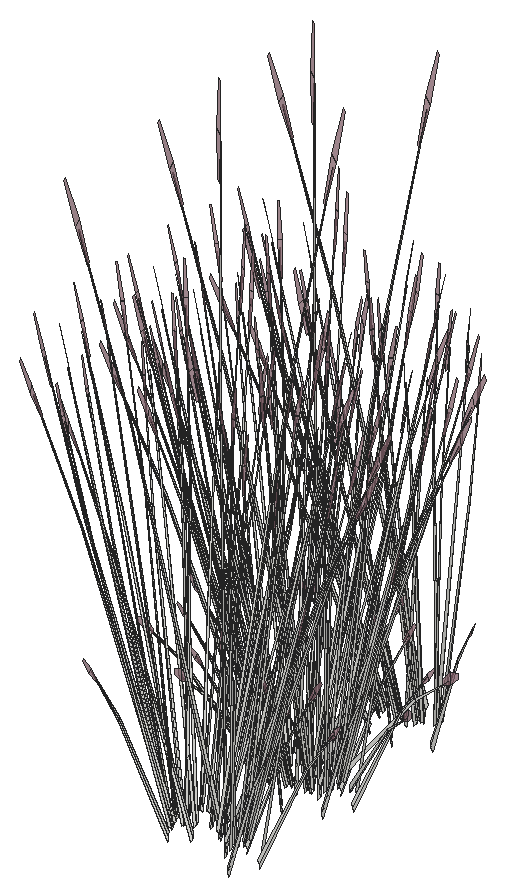
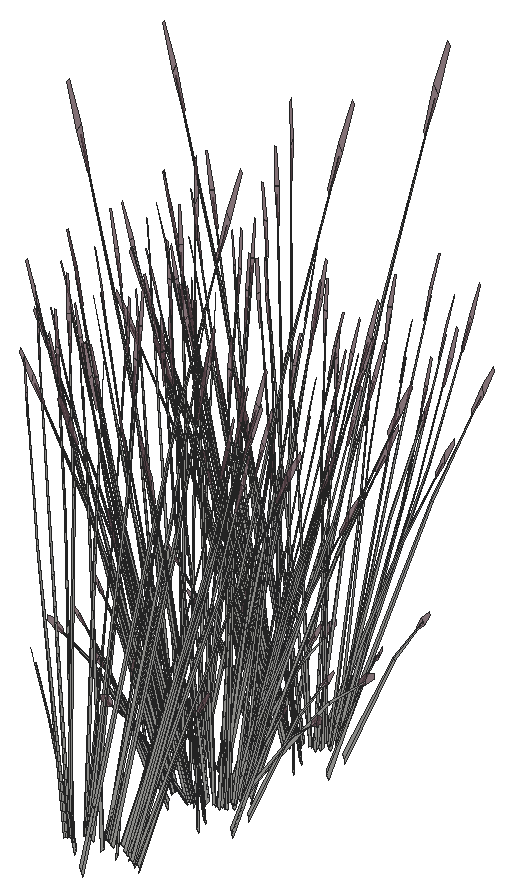
# SketchUp Ruby script. Lengths in inches.
U = 1.inch
M = Sketchup.active_model
def pt(a) = Geom::Point3d.new(a.map { |v| v * U })
def face(e, loops, mat)
  f = e.add_face(loops[0].map { |a| pt(a) })
  loops[1..].each { |l| e.add_face(l.map { |a| pt(a) }).erase! }
  f.material = f.back_material = mat if mat
  f
end
# faces: each face lists its corners as indices into pts; further lists are holes
def faces(e, pts, list, mat = nil) = list.each { |f| face(e, (f[0].is_a?(Array) ? f : [f]).map { |l| l.map { |i| pts[i] } }, mat) }
# xy, xz, yz: faces in a plane at the given z, y or x. An outline is a flat list of corners, or four numbers for a rectangle; further outlines are holes
def ring(l) = l.size == 4 ? [[l[0], l[1]], [l[2], l[1]], [l[2], l[3]], [l[0], l[3]]] : l.each_slice(2).to_a
def flat(e, list, mat, &to3) = list.each { |f| face(e, (f[0].is_a?(Array) ? f : [f]).map { |l| ring(l).map { |u, v| to3.(u, v) } }, mat) }
def xy(e, z, list, mat = nil) = flat(e, list, mat) { |x, y| [x, y, z] }
def xz(e, y, list, mat = nil) = flat(e, list, mat) { |x, z| [x, y, z] }
def yz(e, x, list, mat = nil) = flat(e, list, mat) { |y, z| [x, y, z] }
def lines(e, pts, list) = list.each { |a, b| e.add_line(pt(pts[a]), pt(pts[b])) }
# prism: a flat outline (further loops are holes) pulled along v
def prism(e, loops, v, mat = nil)
  f = face(e, loops, mat); d = Geom::Vector3d.new(v.map { |x| x * U })
  f.pushpull(f.normal.samedirection?(d) ? d.length : -d.length)
end
def box(e, o, s, mat = nil) = prism(e, [[o, [o[0] + s[0], o[1], o[2]], [o[0] + s[0], o[1] + s[1], o[2]], [o[0], o[1] + s[1], o[2]]]], [0, 0, s[2]], mat)
def at(x, y, z, deg = 0) = Geom::Transformation.translation(pt([x, y, z])) * Geom::Transformation.rotation(ORIGIN, Z_AXIS, deg.degrees)
def axes(o, x, y, z) = Geom::Transformation.new([*x, 0, *y, 0, *z, 0, *pt(o).to_a, 1])
def part(name) = M.definitions.add(name)
# library, detail: a bought-in or finely detailed component or shape, given as its bounding box
def library(name, o, s) = part(name).tap { |d| box(d.entities, o, s) }
def detail(e, o, s) = box(e.add_group.entities, o, s)
def put(e, d, t, mat = nil) = e.add_instance(d, t).tap { |i| i.material = mat if mat }
def group(e, t, mat = nil) = e.add_group.tap { |g| g.transformation = t; g.material = mat if mat }.entities
root = M.entities
M.materials.add("LightPink_Translucent").color = [144, 107, 117]
M.materials["LightPink_Translucent"].alpha = 0.75
c1 = part("blade")
p = [[2.15,0.21,22],[0,0.17,0],[0.09,0.45,0],[2.18,0.31,22],[2.29,0.31,22],[0.38,0.45,0],
  [2.48,0.24,33],[2.49,0.24,33],[2.48,0.22,33]]
faces(c1.entities,p,[[0,1,2,3],[4,5,2,3],[6,3,4,7],[8,0,3,6]])
c2 = part("seeds")
p = [[0.3,-0.1,1.38],[-0.01,-0.03,1.59],[-0.01,-0.03,0.03],[0.14,-0.07,-0.07],[0.29,-0.03,3],[0.15,0.01,3.11]]
faces(c2.entities,p,[[0,1,2,3],[1,0,4,5]],"LightPink_Translucent")
c3 = part("blade with seeds")
put(c3.entities,c1,at(0,0,0))
put(c3.entities,c2,axes([2.4,0.25,30.99],[1.5799,-0.05474,1.17369],[-0.12525,1.92788,0.29478],[-0.07173,-0.02425,1.56792]))
put(root,c3,axes([335.76,404.49,52.14],[-0.12971,-0.3568,-0.45151],[0.49122,-0.06241,-0.34973],[0.14077,-0.09583,0.86392]))
put(root,c3,axes([335.99,404.74,52.45],[-0.46706,-0.21546,-0.10745],[0.26908,-0.31203,-0.59638],[0.13196,-0.10846,0.90619]))
put(root,c3,axes([334.06,405.92,50.9375],[0.43633,0.15757,1.33654],[-0.42745,0.33945,0.52853],[-0.19146,-0.20119,1.12046]))
put(root,c3,axes([336.36,403.78,50.44],[-0.16818,0.19891,1.01491],[-0.14456,-0.26725,0.74569],[0.1389,-0.06697,0.22354]))
put(root,c3,axes([336.12,404.52,52],[0.43951,-0.05584,-0.31292],[0.11606,0.31924,0.40398],[0.12595,-0.08575,0.77298]))
put(root,c3,axes([331.85,404.09,52],[-0.28729,-0.24465,-0.31292],[0.32804,-0.23159,0.40398],[-0.16667,-0.03524,0.77298]))
put(root,c3,axes([332.15,404.25,52.4],[-0.50473,-0.00941,-0.62776],[0.0339,-0.39618,0.07576],[-0.21383,-0.04181,0.88802]))
put(root,c3,axes([331.98,404.33,52.14],[-0.36663,0.25884,-0.45151],[-0.32109,-0.27343,-0.34973],[-0.18628,-0.03938,0.86392]))
put(root,c3,axes([331.16,404.67,50.44],[0.32236,-0.02796,1.01491],[-0.20448,0.24636,0.74569],[-0.1593,-0.03696,0.22354]))
put(root,c3,axes([332.18,404.06,52.45],[-0.02704,0.39739,-0.10745],[-0.51189,-0.01086,-0.59638],[-0.19715,-0.0276,0.90619]))
put(root,c3,axes([336.01,405.58,52.45],[-0.25405,-0.35383,-0.10745],[0.45089,-0.17388,-0.59638],[0.19001,-0.04668,0.90619]))
put(root,c3,axes([335.98,405.28,52.14],[0.13679,-0.35544,-0.45151],[0.46898,0.12183,-0.34973],[0.18882,-0.03259,0.86392]))
put(root,c3,axes([331.52,404.61,51.43],[0.20943,-0.00885,1.51428],[-0.13893,0.38357,0.12244],[-0.29846,-0.02372,0.64734]))
put(root,c3,axes([335.9,405.41,52.4],[0.44368,-0.17257,-0.62776],[0.24726,0.35524,0.07576],[0.21437,-0.04035,0.88802]))
put(root,c3,axes([336.27,405.44,52],[0.41962,0.10901,-0.31292],[-0.12239,0.31802,0.40398],[0.16894,-0.02916,0.77298]))
put(root,c3,axes([331.34,404.93,52],[-0.41962,-0.10901,-0.31292],[0.12239,-0.31802,0.40398],[-0.16894,0.02916,0.77298]))
put(root,c3,axes([335.13,405.05,51.43],[-0.20943,0.00885,1.51428],[0.13893,-0.38357,0.12244],[0.29846,0.02372,0.64734]))
put(root,c3,axes([332.62,404.88,50.95],[0.14352,-0.05653,1.56454],[0.04949,0.39467,0.12244],[-0.31087,0.05237,0.55918]))
put(root,c3,axes([337.16,405.51,50.44],[-0.31197,0.06451,1.01491],[0.14684,-0.26661,0.74569],[0.1655,0.01824,0.22354]))
put(root,c3,axes([331.63,405.1,52.14],[-0.13679,0.35544,-0.45151],[-0.46898,-0.12183,-0.34973],[-0.18882,0.03259,0.86392]))
put(root,c3,axes([331.61,404.79,52.45],[0.25405,0.35383,-0.10745],[-0.45089,0.17388,-0.59638],[-0.19001,0.04668,0.90619]))
put(root,c3,axes([336.62,406.33,51.47],[-0.09664,-0.32847,-0.03085],[0.45676,-0.07551,-0.13989],[0.09538,0.02082,0.4614]))
put(root,c3,axes([335.4375,406.32,52.45],[0.02704,-0.39739,-0.10745],[0.51189,0.01086,-0.59638],[0.19715,0.0276,0.90619]))
put(root,c3,axes([331.61,405.28,51.43],[0.17519,-0.08265,1.51428],[0.14749,0.38193,0.12244],[-0.27504,0.08632,0.64734]))
put(root,c3,axes([335.46,406.125,52.4],[0.50473,0.00941,-0.62776],[-0.0339,0.39618,0.07576],[0.21383,0.04181,0.88802]))
put(root,c3,axes([330.7,406.62,50.44],[0.21042,-0.1771,1.01491],[0.08303,0.28036,0.74569],[-0.15207,0.0502,0.22354]))
put(root,c3,axes([335.77,406.29,52],[0.28729,0.24465,-0.31292],[-0.32804,0.23159,0.40398],[0.16667,0.03524,0.77298]))
put(root,c3,axes([331.49,405.85,52],[-0.43951,0.05584,-0.31292],[-0.11606,-0.31924,0.40398],[-0.12595,0.08575,0.77298]))
put(root,c3,axes([334.73,405.66,51.43],[-0.18755,-0.06732,1.51428],[0.38813,-0.28243,0.12244],[0.24191,0.12741,0.64734]))
put(root,c3,axes([334.77,404.78,51.95],[-0.4363,-0.20303,1.22187],[0.46069,-0.31611,0.5272],[0.14077,0.1905,1.18105]))
put(root,c3,axes([331.625,405.63,52.45],[0.46706,0.21546,-0.10745],[-0.26908,0.31203,-0.59638],[-0.13196,0.10846,0.90619]))
put(root,c3,axes([335.43,406.43,50.44],[-0.28429,-0.11236,1.01491],[0.36709,-0.11416,0.74569],[0.09901,0.0967,0.22354]))
put(root,c3,axes([334.43,406.75,52.45],[0.30087,-0.33447,-0.10745],[0.43572,0.19269,-0.59638],[0.15146,0.0945,0.90619]))
put(root,c3,axes([332.25,405.54,51.43],[0.12611,-0.12006,1.51428],[0.31843,0.32408,0.12244],[-0.2184,0.14759,0.64734]))
put(root,c3,axes([331.86,405.89,52.14],[0.12971,0.3568,-0.45151],[-0.49122,0.06241,-0.34973],[-0.14077,0.09583,0.86392]))
put(root,c3,axes([334.74,405.17,50.51],[-0.01379,-0.36791,1.24828],[0.62424,0.09537,0.52853],[-0.14764,0.20132,1.17828]))
put(root,c3,axes([334.79,406.58,52.14],[0.49824,-0.09289,-0.45151],[0.08716,0.35177,-0.34973],[0.13382,0.10081,0.86392]))
put(root,c3,axes([332.69,412.0625,51.43],[0.11542,0.12546,1.51428],[-0.53333,0.10562,0.12244],[-0.12054,-0.19696,0.64734]))
put(root,c3,axes([333.57,411.23,52.17],[-0.07723,-0.05479,1.54581],[-0.51538,0.03473,-0.24447],[-0.08225,-0.13104,0.12397]))
put(root,c3,axes([332.16,405.83,51.43],[0.09401,-0.13431,1.51428],[0.3944,0.27795,0.12244],[-0.17792,0.17323,0.64734]))
put(root,c3,axes([334.11,412.16,52.4],[-0.24099,-0.31773,-0.62776],[0.49607,-0.17707,0.07576],[-0.05635,-0.15352,0.88802]))
put(root,c3,axes([332.27,406.59,52],[-0.34164,0.20573,-0.31292],[-0.3234,-0.23491,0.40398],[-0.04921,0.11936,0.77298]))
put(root,c3,axes([333.25,406.76,52.45],[0.49409,-0.18193,-0.10745],[0.24281,0.32289,-0.59638],[0.06519,0.13607,0.90619]))
put(root,c3,axes([332.48,407.39,50.44],[-0.01307,-0.23234,1.01491],[0.32652,0.16572,0.74569],[-0.06422,0.11074,0.22354]))
put(root,c3,axes([335.12,412.47,52.4],[0.01314,-0.36145,-0.62776],[0.55324,0.02428,0.07576],[0.05838,-0.15313,0.88802]))
put(root,c3,axes([335.89,411.9,52.17],[-0.00487,-0.07777,1.54581],[-0.41166,-0.22476,-0.24447],[0.06364,-0.13625,0.12397]))
put(root,c3,axes([334.16,411.89,52],[0.15222,-0.30049,-0.31292],[0.44409,0.08764,0.40398],[-0.04072,-0.12098,0.77298]))
put(root,c3,axes([334.5,412.29,51.43],[-0.09401,0.13431,1.51428],[-0.3944,-0.27795,0.12244],[0.17792,-0.17323,0.64734]))
put(root,c3,axes([332.61,406.49,52.42],[0.36145,0.26255,-0.50118],[-0.38183,0.22994,-0.3882],[-0.055,0.1334,0.95895]))
put(root,c3,axes([333.68,406.75,52.14],[0.49634,0.09796,-0.45151],[-0.17013,0.33585,-0.34973],[0.04551,0.13522,0.86392]))
put(root,c3,axes([333.96,406.05,51.43],[-0.11542,-0.12546,1.51428],[0.53333,-0.10562,0.12244],[0.12054,0.19696,0.64734]))
put(root,c3,axes([333.93,412.09,52.14],[-0.49634,-0.09796,-0.45151],[0.17013,-0.33585,-0.34973],[-0.04551,-0.13522,0.86392]))
put(root,c3,axes([334.24,411.25,50.44],[0.06477,0.22786,1.01491],[-0.35932,-0.1262,0.74569],[0.03867,-0.11667,0.22354]))
put(root,c3,axes([335.01,412.35,52.14],[-0.36145,-0.26255,-0.45151],[0.38183,-0.22994,-0.34973],[0.055,-0.1334,0.86392]))
put(root,c3,axes([333.45,406.95,52],[-0.15222,0.30049,-0.31292],[-0.44409,-0.08764,0.40398],[0.04072,0.12098,0.77298]))
put(root,c3,axes([332.49,406.375,52.72],[-0.01314,0.36145,-0.69681],[-0.55324,-0.02428,0.08409],[-0.05838,0.15313,0.9857]))
put(root,c3,axes([333.02,406.12,51.43],[-0.01236,-0.14998,1.51428],[0.53562,0.09949,0.12244],[-0.03313,0.21373,0.64734]))
put(root,c3,axes([334.36,412.08,52.45],[-0.49409,0.18193,-0.10745],[-0.24281,-0.32289,-0.59638],[-0.06519,-0.13607,0.90619]))
put(root,c3,axes([335.38,412.49,52.45],[-0.55492,-0.01936,-0.10745],[0.01517,-0.36657,-0.59638],[0.03855,-0.14118,0.90619]))
put(root,c3,axes([335.35,412.25,52],[0.34164,-0.20573,-0.31292],[0.3234,0.23491,0.40398],[0.04921,-0.11936,0.77298]))
put(root,c3,axes([332.39,411.53,50.44],[0.26338,0.136,1.01491],[-0.38358,0.08175,0.74569],[-0.08207,-0.10452,0.22354]))
put(root,c3,axes([333.03,412.25,52.4],[-0.43054,-0.18887,-0.62776],[0.30598,-0.33097,0.07576],[-0.15599,-0.11277,0.88802]))
put(root,c3,axes([332.88,412,52],[-0.07798,-0.31474,-0.31292],[0.44579,-0.08311,0.40398],[-0.11974,-0.09019,0.77298]))
put(root,c3,axes([333.5,406.68,52.4],[0.24099,0.31773,-0.62776],[-0.49607,0.17707,0.07576],[0.05635,0.15352,0.88802]))
put(root,c3,axes([331.92,412.46,51.43],[0.18755,0.06732,1.51428],[-0.38813,0.28243,0.12244],[-0.24191,-0.12741,0.64734]))
put(root,c3,axes([332.83,412.26,52.14],[-0.49824,0.09289,-0.45151],[-0.08716,-0.35177,-0.34973],[-0.13382,-0.10081,0.86392]))
put(root,c3,axes([332.31,406.88,50.97],[0.01109,-0.20172,1.3638],[0.49896,0.10655,0.18846],[-0.04323,0.21498,0.64398]))
put(root,c3,axes([335.77,413.1,52.4],[0.26374,-0.30832,-0.62776],[0.46217,0.21911,0.07576],[0.15748,-0.11171,0.88802]))
put(root,c3,axes([335.76,412.95,52.14],[-0.12971,-0.3568,-0.45151],[0.49122,-0.06241,-0.34973],[0.14077,-0.09583,0.86392]))
put(root,c3,axes([331.88,411.84,52.17],[-0.10864,-0.00276,1.54581],[-0.34587,0.27582,-0.24447],[-0.18454,-0.05636,0.12397]))
put(root,c3,axes([335.99,413.21,52.45],[-0.46706,-0.21546,-0.10745],[0.26908,-0.31203,-0.59638],[0.13196,-0.10846,0.90619]))
put(root,c3,axes([334.06,414.38,50.9375],[0.43633,0.15757,1.33654],[-0.42745,0.33945,0.52853],[-0.19146,-0.20119,1.12046]))
put(root,c3,axes([336.36,412.24,50.44],[-0.16818,0.19891,1.01491],[-0.14456,-0.26725,0.74569],[0.1389,-0.06697,0.22354]))
put(root,c3,axes([336.12,412.99,52],[0.43951,-0.05584,-0.31292],[0.11606,0.31924,0.40398],[0.12595,-0.08575,0.77298]))
put(root,c3,axes([331.85,412.55,52],[-0.28729,-0.24465,-0.31292],[0.32804,-0.23159,0.40398],[-0.16667,-0.03524,0.77298]))
put(root,c3,axes([332.15,412.71,52.4],[-0.50473,-0.00941,-0.62776],[0.0339,-0.39618,0.07576],[-0.21383,-0.04181,0.88802]))
put(root,c3,axes([337.39,413.49,52.17],[0.07006,-0.05952,1.54581],[-0.08968,-0.3651,-0.24447],[0.1758,-0.06922,0.12397]))
put(root,c3,axes([331.98,412.8,52.14],[-0.36663,0.25884,-0.45151],[-0.32109,-0.27343,-0.34973],[-0.18628,-0.03938,0.86392]))
put(root,c3,axes([331.16,413.14,50.44],[0.32236,-0.02796,1.01491],[-0.20448,0.24636,0.74569],[-0.1593,-0.03696,0.22354]))
put(root,c3,axes([332.18,412.52,52.45],[-0.02704,0.39739,-0.10745],[-0.51189,-0.01086,-0.59638],[-0.19715,-0.0276,0.90619]))
put(root,c3,axes([336.01,414.05,52.45],[-0.25405,-0.35383,-0.10745],[0.45089,-0.17388,-0.59638],[0.19001,-0.04668,0.90619]))
put(root,c3,axes([335.98,413.75,52.14],[0.13679,-0.35544,-0.45151],[0.46898,0.12183,-0.34973],[0.18882,-0.03259,0.86392]))
put(root,c3,axes([331.52,413.07,51.43],[0.20943,-0.00885,1.51428],[-0.13893,0.38357,0.12244],[-0.29846,-0.02372,0.64734]))
put(root,c3,axes([335.9,413.875,52.4],[0.44368,-0.17257,-0.62776],[0.24726,0.35524,0.07576],[0.21437,-0.04035,0.88802]))
put(root,c3,axes([336.27,413.91,52],[0.41962,0.10901,-0.31292],[-0.12239,0.31802,0.40398],[0.16894,-0.02916,0.77298]))
put(root,c3,axes([331.34,413.4,52],[-0.41962,-0.10901,-0.31292],[0.12239,-0.31802,0.40398],[-0.16894,0.02916,0.77298]))
put(root,c3,axes([335.13,413.51,51.43],[-0.20943,0.00885,1.51428],[0.13893,-0.38357,0.12244],[0.29846,0.02372,0.64734]))
put(root,c3,axes([332.62,413.35,50.95],[0.14352,-0.05653,1.56454],[0.04949,0.39467,0.12244],[-0.31087,0.05237,0.55918]))
put(root,c3,axes([337.16,413.97,50.44],[-0.31197,0.06451,1.01491],[0.14684,-0.26661,0.74569],[0.1655,0.01824,0.22354]))
put(root,c3,axes([331.08,413.61,52.17],[-0.08245,0.05073,1.54581],[0.00701,0.37067,-0.24447],[-0.18899,0.0482,0.12397]))
put(root,c3,axes([331.63,413.5625,52.14],[-0.13679,0.35544,-0.45151],[-0.46898,-0.12183,-0.34973],[-0.18882,0.03259,0.86392]))
put(root,c3,axes([331.61,413.26,52.45],[0.25405,0.35383,-0.10745],[-0.45089,0.17388,-0.59638],[-0.19001,0.04668,0.90619]))
put(root,c3,axes([336.62,414.79,51.47],[-0.09664,-0.32847,-0.03085],[0.45676,-0.07551,-0.13989],[0.09538,0.02082,0.4614]))
put(root,c3,axes([335.4375,414.78,52.45],[0.02704,-0.39739,-0.10745],[0.51189,0.01086,-0.59638],[0.19715,0.0276,0.90619]))
put(root,c3,axes([335.88,414.55,52.17],[0.10831,-0.00661,1.54581],[0.29709,-0.30358,-0.24447],[0.19266,0.04007,0.12397]))
put(root,c3,axes([331.61,413.75,51.43],[0.17519,-0.08265,1.51428],[0.14749,0.38193,0.12244],[-0.27504,0.08632,0.64734]))
put(root,c3,axes([335.46,414.59,52.4],[0.50473,0.00941,-0.62776],[-0.0339,0.39618,0.07576],[0.21383,0.04181,0.88802]))
put(root,c3,axes([330.7,415.08,50.44],[0.21042,-0.1771,1.01491],[0.08303,0.28036,0.74569],[-0.15207,0.0502,0.22354]))
put(root,c3,axes([335.77,414.76,52],[0.28729,0.24465,-0.31292],[-0.32804,0.23159,0.40398],[0.16667,0.03524,0.77298]))
put(root,c3,axes([331.49,414.32,52],[-0.43951,0.05584,-0.31292],[-0.11606,-0.31924,0.40398],[-0.12595,0.08575,0.77298]))
put(root,c3,axes([334.73,414.13,51.43],[-0.18755,-0.06732,1.51428],[0.38813,-0.28243,0.12244],[0.24191,0.12741,0.64734]))
put(root,c3,axes([334.77,413.24,51.95],[-0.4363,-0.20303,1.22187],[0.46069,-0.31611,0.5272],[0.14077,0.1905,1.18105]))
put(root,c3,axes([331.625,414.1,52.45],[0.46706,0.21546,-0.10745],[-0.26908,0.31203,-0.59638],[-0.13196,0.10846,0.90619]))
put(root,c3,axes([335.43,414.9,50.44],[-0.28429,-0.11236,1.01491],[0.36709,-0.11416,0.74569],[0.09901,0.0967,0.22354]))
put(root,c3,axes([334.43,415.22,52.45],[0.30087,-0.33447,-0.10745],[0.43572,0.19269,-0.59638],[0.15146,0.0945,0.90619]))
put(root,c3,axes([332.25,414,51.43],[0.12611,-0.12006,1.51428],[0.31843,0.32408,0.12244],[-0.2184,0.14759,0.64734]))
put(root,c3,axes([331.86,414.36,52.14],[0.12971,0.3568,-0.45151],[-0.49122,0.06241,-0.34973],[-0.14077,0.09583,0.86392]))
put(root,c3,axes([334.74,413.63,50.51],[-0.01379,-0.36791,1.24828],[0.62424,0.09537,0.52853],[-0.14764,0.20132,1.17828]))
put(root,c3,axes([334.79,415.05,52.14],[0.49824,-0.09289,-0.45151],[0.08716,0.35177,-0.34973],[0.13382,0.10081,0.86392]))
put(root,c3,axes([332.16,414.3,51.43],[0.09401,-0.13431,1.51428],[0.3944,0.27795,0.12244],[-0.17792,0.17323,0.64734]))
put(root,c3,axes([332.27,415.06,52],[-0.34164,0.20573,-0.31292],[-0.3234,-0.23491,0.40398],[-0.04921,0.11936,0.77298]))
put(root,c3,axes([331.09,415,52.17],[-0.01255,0.07733,1.54581],[0.35618,0.269,-0.24447],[-0.09325,0.12721,0.12397]))
put(root,c3,axes([333.25,415.23,52.45],[0.49409,-0.18193,-0.10745],[0.24281,0.32289,-0.59638],[0.06519,0.13607,0.90619]))
put(root,c3,axes([332.48,415.86,50.44],[-0.01307,-0.23234,1.01491],[0.32652,0.16572,0.74569],[-0.06422,0.11074,0.22354]))
put(root,c3,axes([332.61,414.96,52.42],[0.36145,0.26255,-0.50118],[-0.38183,0.22994,-0.3882],[-0.055,0.1334,0.95895]))
put(root,c3,axes([333.68,415.21,52.14],[0.49634,0.09796,-0.45151],[-0.17013,0.33585,-0.34973],[0.04551,0.13522,0.86392]))
put(root,c3,axes([333.96,414.52,51.43],[-0.11542,-0.12546,1.51428],[0.53333,-0.10562,0.12244],[0.12054,0.19696,0.64734]))
put(root,c3,axes([333.45,415.42,52],[-0.15222,0.30049,-0.31292],[-0.44409,-0.08764,0.40398],[0.04072,0.12098,0.77298]))
put(root,c3,axes([332.49,414.84,52.72],[-0.01314,0.36145,-0.69681],[-0.55324,-0.02428,0.08409],[-0.05838,0.15313,0.9857]))
put(root,c3,axes([333.02,414.58,51.43],[-0.01236,-0.14998,1.51428],[0.53562,0.09949,0.12244],[-0.03313,0.21373,0.64734]))
put(root,c3,axes([333.5,415.15,52.4],[0.24099,0.31773,-0.62776],[-0.49607,0.17707,0.07576],[0.05635,0.15352,0.88802]))
put(root,c3,axes([333.14,415.95,52.17],[0.064,0.06292,1.54581],[0.51651,0.02472,-0.24447],[0.05194,0.13877,0.12397]))
put(root,c3,axes([332.69,421.96,51.43],[0.11542,0.12546,1.51428],[-0.53333,0.10562,0.12244],[-0.12054,-0.19696,0.64734]))
put(root,c3,axes([334.11,422.06,52.4],[-0.24099,-0.31773,-0.62776],[0.49607,-0.17707,0.07576],[-0.05635,-0.15352,0.88802]))
put(root,c3,axes([332.31,415.35,50.97],[0.01109,-0.20172,1.3638],[0.49896,0.10655,0.18846],[-0.04323,0.21498,0.64398]))
put(root,c3,axes([335.12,422.37,52.4],[0.01314,-0.36145,-0.62776],[0.55324,0.02428,0.07576],[0.05838,-0.15313,0.88802]))
put(root,c3,axes([334.16,421.79,52],[0.15222,-0.30049,-0.31292],[0.44409,0.08764,0.40398],[-0.04072,-0.12098,0.77298]))
put(root,c3,axes([334.5,422.18,51.43],[-0.09401,0.13431,1.51428],[-0.3944,-0.27795,0.12244],[0.17792,-0.17323,0.64734]))
put(root,c3,axes([333.93,421.99,52.14],[-0.49634,-0.09796,-0.45151],[0.17013,-0.33585,-0.34973],[-0.04551,-0.13522,0.86392]))
put(root,c3,axes([334.24,421.15,50.44],[0.06477,0.22786,1.01491],[-0.35932,-0.1262,0.74569],[0.03867,-0.11667,0.22354]))
put(root,c3,axes([335.01,422.25,52.14],[-0.36145,-0.26255,-0.45151],[0.38183,-0.22994,-0.34973],[0.055,-0.1334,0.86392]))
put(root,c3,axes([334.36,421.98,52.45],[-0.49409,0.18193,-0.10745],[-0.24281,-0.32289,-0.59638],[-0.06519,-0.13607,0.90619]))
put(root,c3,axes([335.38,422.38,52.45],[-0.55492,-0.01936,-0.10745],[0.01517,-0.36657,-0.59638],[0.03855,-0.14118,0.90619]))
put(root,c3,axes([335.35,422.15,52],[0.34164,-0.20573,-0.31292],[0.3234,0.23491,0.40398],[0.04921,-0.11936,0.77298]))
put(root,c3,axes([332.39,421.42,50.44],[0.26338,0.136,1.01491],[-0.38358,0.08175,0.74569],[-0.08207,-0.10452,0.22354]))
put(root,c3,axes([333.03,422.15,52.4],[-0.43054,-0.18887,-0.62776],[0.30598,-0.33097,0.07576],[-0.15599,-0.11277,0.88802]))
put(root,c3,axes([332.88,421.9,52],[-0.07798,-0.31474,-0.31292],[0.44579,-0.08311,0.40398],[-0.11974,-0.09019,0.77298]))
put(root,c3,axes([331.92,422.35,51.43],[0.18755,0.06732,1.51428],[-0.38813,0.28243,0.12244],[-0.24191,-0.12741,0.64734]))
put(root,c3,axes([332.83,422.16,52.14],[-0.49824,0.09289,-0.45151],[-0.08716,-0.35177,-0.34973],[-0.13382,-0.10081,0.86392]))
put(root,c3,axes([335.77,422.99,52.4],[0.26374,-0.30832,-0.62776],[0.46217,0.21911,0.07576],[0.15748,-0.11171,0.88802]))
put(root,c3,axes([335.76,422.85,52.14],[-0.12971,-0.3568,-0.45151],[0.49122,-0.06241,-0.34973],[0.14077,-0.09583,0.86392]))
put(root,c3,axes([335.99,423.11,52.45],[-0.46706,-0.21546,-0.10745],[0.26908,-0.31203,-0.59638],[0.13196,-0.10846,0.90619]))
put(root,c3,axes([334.06,424.28,50.9375],[0.43633,0.15757,1.33654],[-0.42745,0.33945,0.52853],[-0.19146,-0.20119,1.12046]))
put(root,c3,axes([336.36,422.14,50.44],[-0.16818,0.19891,1.01491],[-0.14456,-0.26725,0.74569],[0.1389,-0.06697,0.22354]))
put(root,c3,axes([336.12,422.89,52],[0.43951,-0.05584,-0.31292],[0.11606,0.31924,0.40398],[0.12595,-0.08575,0.77298]))
put(root,c3,axes([331.85,422.45,52],[-0.28729,-0.24465,-0.31292],[0.32804,-0.23159,0.40398],[-0.16667,-0.03524,0.77298]))
put(root,c3,axes([332.15,422.61,52.4],[-0.50473,-0.00941,-0.62776],[0.0339,-0.39618,0.07576],[-0.21383,-0.04181,0.88802]))
put(root,c3,axes([331.98,422.69,52.14],[-0.36663,0.25884,-0.45151],[-0.32109,-0.27343,-0.34973],[-0.18628,-0.03938,0.86392]))
